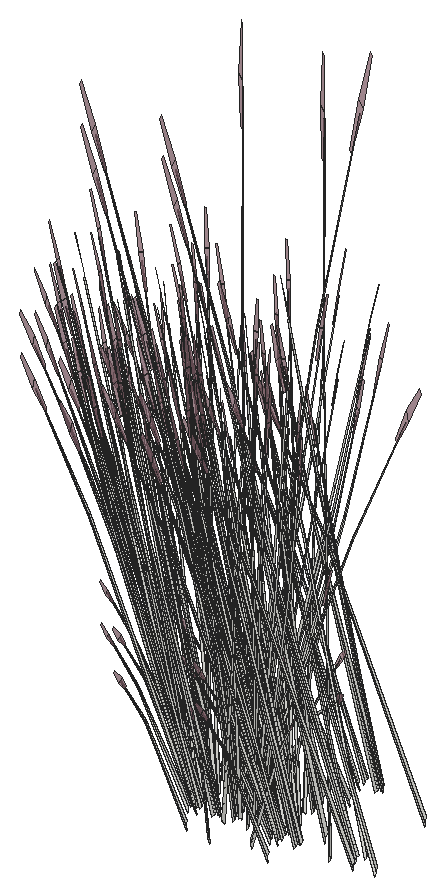
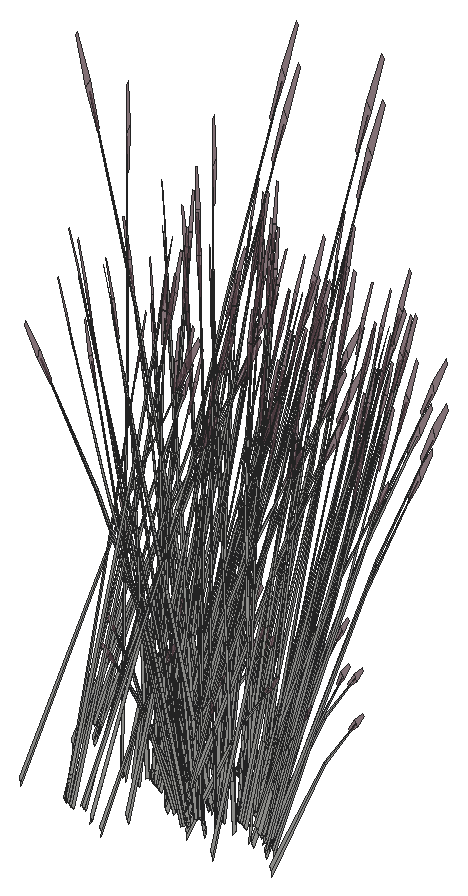
# SketchUp Ruby script. Lengths in inches.
U = 1.inch
M = Sketchup.active_model
def pt(a) = Geom::Point3d.new(a.map { |v| v * U })
def face(e, loops, mat)
  f = e.add_face(loops[0].map { |a| pt(a) })
  loops[1..].each { |l| e.add_face(l.map { |a| pt(a) }).erase! }
  f.material = f.back_material = mat if mat
  f
end
# faces: each face lists its corners as indices into pts; further lists are holes
def faces(e, pts, list, mat = nil) = list.each { |f| face(e, (f[0].is_a?(Array) ? f : [f]).map { |l| l.map { |i| pts[i] } }, mat) }
# xy, xz, yz: faces in a plane at the given z, y or x. An outline is a flat list of corners, or four numbers for a rectangle; further outlines are holes
def ring(l) = l.size == 4 ? [[l[0], l[1]], [l[2], l[1]], [l[2], l[3]], [l[0], l[3]]] : l.each_slice(2).to_a
def flat(e, list, mat, &to3) = list.each { |f| face(e, (f[0].is_a?(Array) ? f : [f]).map { |l| ring(l).map { |u, v| to3.(u, v) } }, mat) }
def xy(e, z, list, mat = nil) = flat(e, list, mat) { |x, y| [x, y, z] }
def xz(e, y, list, mat = nil) = flat(e, list, mat) { |x, z| [x, y, z] }
def yz(e, x, list, mat = nil) = flat(e, list, mat) { |y, z| [x, y, z] }
def lines(e, pts, list) = list.each { |a, b| e.add_line(pt(pts[a]), pt(pts[b])) }
# prism: a flat outline (further loops are holes) pulled along v
def prism(e, loops, v, mat = nil)
  f = face(e, loops, mat); d = Geom::Vector3d.new(v.map { |x| x * U })
  f.pushpull(f.normal.samedirection?(d) ? d.length : -d.length)
end
def box(e, o, s, mat = nil) = prism(e, [[o, [o[0] + s[0], o[1], o[2]], [o[0] + s[0], o[1] + s[1], o[2]], [o[0], o[1] + s[1], o[2]]]], [0, 0, s[2]], mat)
def at(x, y, z, deg = 0) = Geom::Transformation.translation(pt([x, y, z])) * Geom::Transformation.rotation(ORIGIN, Z_AXIS, deg.degrees)
def axes(o, x, y, z) = Geom::Transformation.new([*x, 0, *y, 0, *z, 0, *pt(o).to_a, 1])
def part(name) = M.definitions.add(name)
# library, detail: a bought-in or finely detailed component or shape, given as its bounding box
def library(name, o, s) = part(name).tap { |d| box(d.entities, o, s) }
def detail(e, o, s) = box(e.add_group.entities, o, s)
def put(e, d, t, mat = nil) = e.add_instance(d, t).tap { |i| i.material = mat if mat }
def group(e, t, mat = nil) = e.add_group.tap { |g| g.transformation = t; g.material = mat if mat }.entities
root = M.entities
M.materials.add("LightPink_Translucent").color = [144, 107, 117]
M.materials["LightPink_Translucent"].alpha = 0.75
c1 = part("blade")
p = [[2.15,0.21,22],[0,0.17,0],[0.09,0.45,0],[2.18,0.31,22],[2.29,0.31,22],[0.38,0.45,0],
  [2.48,0.24,33],[2.49,0.24,33],[2.48,0.22,33]]
faces(c1.entities,p,[[0,1,2,3],[4,5,2,3],[6,3,4,7],[8,0,3,6]])
c2 = part("seeds")
p = [[0.3,-0.1,1.38],[-0.01,-0.03,1.59],[-0.01,-0.03,0.03],[0.14,-0.07,-0.07],[0.29,-0.03,3],[0.15,0.01,3.11]]
faces(c2.entities,p,[[0,1,2,3],[1,0,4,5]],"LightPink_Translucent")
c3 = part("blade with seeds")
put(c3.entities,c1,at(0,0,0))
put(c3.entities,c2,axes([2.4,0.25,30.99],[1.5799,-0.05474,1.17369],[-0.12525,1.92788,0.29478],[-0.07173,-0.02425,1.56792]))
put(root,c3,axes([327.44,15.14,51.43],[0.11542,0.12546,1.51428],[-0.53333,0.10562,0.12244],[-0.12054,-0.19696,0.64734]))
put(root,c3,axes([333.1,15.14,51.43],[0.11542,0.12546,1.51428],[-0.53333,0.10562,0.12244],[-0.12054,-0.19696,0.64734]))
put(root,c3,axes([328.86,15.23,52.4],[-0.24099,-0.31773,-0.62776],[0.49607,-0.17707,0.07576],[-0.05635,-0.15352,0.88802]))
put(root,c3,axes([334.52,15.23,52.4],[-0.24099,-0.31773,-0.62776],[0.49607,-0.17707,0.07576],[-0.05635,-0.15352,0.88802]))
put(root,c3,axes([329.86,15.54,52.4],[0.01314,-0.36145,-0.62776],[0.55324,0.02428,0.07576],[0.05838,-0.15313,0.88802]))
put(root,c3,axes([328.91,14.96,52],[0.15222,-0.30049,-0.31292],[0.44409,0.08764,0.40398],[-0.04072,-0.12098,0.77298]))
put(root,c3,axes([329.24,15.36,51.43],[-0.09401,0.13431,1.51428],[-0.3944,-0.27795,0.12244],[0.17792,-0.17323,0.64734]))
put(root,c3,axes([328.68,15.17,52.14],[-0.49634,-0.09796,-0.45151],[0.17013,-0.33585,-0.34973],[-0.04551,-0.13522,0.86392]))
put(root,c3,axes([334.34,15.17,52.14],[-0.49634,-0.09796,-0.45151],[0.17013,-0.33585,-0.34973],[-0.04551,-0.13522,0.86392]))
put(root,c3,axes([328.99,14.33,50.44],[0.06477,0.22786,1.01491],[-0.35932,-0.1262,0.74569],[0.03867,-0.11667,0.22354]))
put(root,c3,axes([329.75,15.42,52.14],[-0.36145,-0.26255,-0.45151],[0.38183,-0.22994,-0.34973],[0.055,-0.1334,0.86392]))
put(root,c3,axes([329.11,15.15,52.45],[-0.49409,0.18193,-0.10745],[-0.24281,-0.32289,-0.59638],[-0.06519,-0.13607,0.90619]))
put(root,c3,axes([334.76,15.15,52.45],[-0.49409,0.18193,-0.10745],[-0.24281,-0.32289,-0.59638],[-0.06519,-0.13607,0.90619]))
put(root,c3,axes([330.13,15.56,52.45],[-0.55492,-0.01936,-0.10745],[0.01517,-0.36657,-0.59638],[0.03855,-0.14118,0.90619]))
put(root,c3,axes([330.09,15.32,52],[0.34164,-0.20573,-0.31292],[0.3234,0.23491,0.40398],[0.04921,-0.11936,0.77298]))
put(root,c3,axes([327.14,14.6,50.44],[0.26338,0.136,1.01491],[-0.38358,0.08175,0.74569],[-0.08207,-0.10452,0.22354]))
put(root,c3,axes([332.8,14.6,50.44],[0.26338,0.136,1.01491],[-0.38358,0.08175,0.74569],[-0.08207,-0.10452,0.22354]))
put(root,c3,axes([327.78,15.32,52.4],[-0.43054,-0.18887,-0.62776],[0.30598,-0.33097,0.07576],[-0.15599,-0.11277,0.88802]))
put(root,c3,axes([333.43,15.32,52.4],[-0.43054,-0.18887,-0.62776],[0.30598,-0.33097,0.07576],[-0.15599,-0.11277,0.88802]))
put(root,c3,axes([327.625,15.07,52],[-0.07798,-0.31474,-0.31292],[0.44579,-0.08311,0.40398],[-0.11974,-0.09019,0.77298]))
put(root,c3,axes([333.28,15.07,52],[-0.07798,-0.31474,-0.31292],[0.44579,-0.08311,0.40398],[-0.11974,-0.09019,0.77298]))
put(root,c3,axes([326.67,15.53,51.43],[0.18755,0.06732,1.51428],[-0.38813,0.28243,0.12244],[-0.24191,-0.12741,0.64734]))
put(root,c3,axes([332.32,15.53,51.43],[0.18755,0.06732,1.51428],[-0.38813,0.28243,0.12244],[-0.24191,-0.12741,0.64734]))
put(root,c3,axes([337.92,15.53,51.43],[0.18755,0.06732,1.51428],[-0.38813,0.28243,0.12244],[-0.24191,-0.12741,0.64734]))
put(root,c3,axes([327.57,15.33,52.14],[-0.49824,0.09289,-0.45151],[-0.08716,-0.35177,-0.34973],[-0.13382,-0.10081,0.86392]))
put(root,c3,axes([333.23,15.33,52.14],[-0.49824,0.09289,-0.45151],[-0.08716,-0.35177,-0.34973],[-0.13382,-0.10081,0.86392]))
put(root,c3,axes([330.52,16.17,52.4],[0.26374,-0.30832,-0.62776],[0.46217,0.21911,0.07576],[0.15748,-0.11171,0.88802]))
put(root,c3,axes([330.5,16.03,52.14],[-0.12971,-0.3568,-0.45151],[0.49122,-0.06241,-0.34973],[0.14077,-0.09583,0.86392]))
put(root,c3,axes([330.74,16.28,52.45],[-0.46706,-0.21546,-0.10745],[0.26908,-0.31203,-0.59638],[0.13196,-0.10846,0.90619]))
put(root,c3,axes([328.81,17.46,50.9375],[0.43633,0.15757,1.33654],[-0.42745,0.33945,0.52853],[-0.19146,-0.20119,1.12046]))
put(root,c3,axes([334.46,17.46,50.9375],[0.43633,0.15757,1.33654],[-0.42745,0.33945,0.52853],[-0.19146,-0.20119,1.12046]))
put(root,c3,axes([331.11,15.32,50.44],[-0.16818,0.19891,1.01491],[-0.14456,-0.26725,0.74569],[0.1389,-0.06697,0.22354]))
put(root,c3,axes([330.87,16.0625,52],[0.43951,-0.05584,-0.31292],[0.11606,0.31924,0.40398],[0.12595,-0.08575,0.77298]))
put(root,c3,axes([326.59,15.625,52],[-0.28729,-0.24465,-0.31292],[0.32804,-0.23159,0.40398],[-0.16667,-0.03524,0.77298]))
put(root,c3,axes([332.25,15.625,52],[-0.28729,-0.24465,-0.31292],[0.32804,-0.23159,0.40398],[-0.16667,-0.03524,0.77298]))
put(root,c3,axes([326.9,15.79,52.4],[-0.50473,-0.00941,-0.62776],[0.0339,-0.39618,0.07576],[-0.21383,-0.04181,0.88802]))
put(root,c3,axes([332.55,15.79,52.4],[-0.50473,-0.00941,-0.62776],[0.0339,-0.39618,0.07576],[-0.21383,-0.04181,0.88802]))
put(root,c3,axes([338.15,15.79,52.4],[-0.50473,-0.00941,-0.62776],[0.0339,-0.39618,0.07576],[-0.21383,-0.04181,0.88802]))
put(root,c3,axes([330.24,18.54,51.43],[0.11542,0.12546,1.51428],[-0.53333,0.10562,0.12244],[-0.12054,-0.19696,0.64734]))
put(root,c3,axes([331.66,18.63,52.4],[-0.24099,-0.31773,-0.62776],[0.49607,-0.17707,0.07576],[-0.05635,-0.15352,0.88802]))
put(root,c3,axes([326.73,15.87,52.14],[-0.36663,0.25884,-0.45151],[-0.32109,-0.27343,-0.34973],[-0.18628,-0.03938,0.86392]))
put(root,c3,axes([332.39,15.87,52.14],[-0.36663,0.25884,-0.45151],[-0.32109,-0.27343,-0.34973],[-0.18628,-0.03938,0.86392]))
put(root,c3,axes([324.42,18.85,51.43],[0.11542,0.12546,1.51428],[-0.53333,0.10562,0.12244],[-0.12054,-0.19696,0.64734]))
put(root,c3,axes([325.9,16.21,50.44],[0.32236,-0.02796,1.01491],[-0.20448,0.24636,0.74569],[-0.1593,-0.03696,0.22354]))
put(root,c3,axes([331.5625,16.21,50.44],[0.32236,-0.02796,1.01491],[-0.20448,0.24636,0.74569],[-0.1593,-0.03696,0.22354]))
put(root,c3,axes([325.84,18.9375,52.4],[-0.24099,-0.31773,-0.62776],[0.49607,-0.17707,0.07576],[-0.05635,-0.15352,0.88802]))
put(root,c3,axes([326.92,15.6,52.45],[-0.02704,0.39739,-0.10745],[-0.51189,-0.01086,-0.59638],[-0.19715,-0.0276,0.90619]))
put(root,c3,axes([332.58,15.6,52.45],[-0.02704,0.39739,-0.10745],[-0.51189,-0.01086,-0.59638],[-0.19715,-0.0276,0.90619]))
put(root,c3,axes([331.7,18.36,52],[0.15222,-0.30049,-0.31292],[0.44409,0.08764,0.40398],[-0.04072,-0.12098,0.77298]))
put(root,c3,axes([326.27,16.14,51.43],[0.20943,-0.00885,1.51428],[-0.13893,0.38357,0.12244],[-0.29846,-0.02372,0.64734]))
put(root,c3,axes([331.93,16.14,51.43],[0.20943,-0.00885,1.51428],[-0.13893,0.38357,0.12244],[-0.29846,-0.02372,0.64734]))
put(root,c3,axes([337.52,16.14,51.43],[0.20943,-0.00885,1.51428],[-0.13893,0.38357,0.12244],[-0.29846,-0.02372,0.64734]))
put(root,c3,axes([331.48,18.57,52.14],[-0.49634,-0.09796,-0.45151],[0.17013,-0.33585,-0.34973],[-0.04551,-0.13522,0.86392]))
put(root,c3,axes([331.78,17.73,50.44],[0.06477,0.22786,1.01491],[-0.35932,-0.1262,0.74569],[0.03867,-0.11667,0.22354]))
put(root,c3,axes([326.84,19.25,52.4],[0.01314,-0.36145,-0.62776],[0.55324,0.02428,0.07576],[0.05838,-0.15313,0.88802]))
put(root,c3,axes([332.55,18.82,52.14],[-0.36145,-0.26255,-0.45151],[0.38183,-0.22994,-0.34973],[0.055,-0.1334,0.86392]))
put(root,c3,axes([325.89,18.67,52],[0.15222,-0.30049,-0.31292],[0.44409,0.08764,0.40398],[-0.04072,-0.12098,0.77298]))
put(root,c3,axes([326.22,19.07,51.43],[-0.09401,0.13431,1.51428],[-0.3944,-0.27795,0.12244],[0.17792,-0.17323,0.64734]))
put(root,c3,axes([325.66,18.875,52.14],[-0.49634,-0.09796,-0.45151],[0.17013,-0.33585,-0.34973],[-0.04551,-0.13522,0.86392]))
put(root,c3,axes([325.97,18.03,50.44],[0.06477,0.22786,1.01491],[-0.35932,-0.1262,0.74569],[0.03867,-0.11667,0.22354]))
put(root,c3,axes([331.9,18.55,52.45],[-0.49409,0.18193,-0.10745],[-0.24281,-0.32289,-0.59638],[-0.06519,-0.13607,0.90619]))
put(root,c3,axes([326.73,19.13,52.14],[-0.36145,-0.26255,-0.45151],[0.38183,-0.22994,-0.34973],[0.055,-0.1334,0.86392]))
put(root,c3,axes([332.93,18.96,52.45],[-0.55492,-0.01936,-0.10745],[0.01517,-0.36657,-0.59638],[0.03855,-0.14118,0.90619]))
put(root,c3,axes([329.9375,18,50.44],[0.26338,0.136,1.01491],[-0.38358,0.08175,0.74569],[-0.08207,-0.10452,0.22354]))
put(root,c3,axes([330.57,18.72,52.4],[-0.43054,-0.18887,-0.62776],[0.30598,-0.33097,0.07576],[-0.15599,-0.11277,0.88802]))
put(root,c3,axes([330.42,18.47,52],[-0.07798,-0.31474,-0.31292],[0.44579,-0.08311,0.40398],[-0.11974,-0.09019,0.77298]))
put(root,c3,axes([326.08,18.86,52.45],[-0.49409,0.18193,-0.10745],[-0.24281,-0.32289,-0.59638],[-0.06519,-0.13607,0.90619]))
put(root,c3,axes([327.11,19.27,52.45],[-0.55492,-0.01936,-0.10745],[0.01517,-0.36657,-0.59638],[0.03855,-0.14118,0.90619]))
put(root,c3,axes([327.07,19.03,52],[0.34164,-0.20573,-0.31292],[0.3234,0.23491,0.40398],[0.04921,-0.11936,0.77298]))
put(root,c3,axes([324.12,18.31,50.44],[0.26338,0.136,1.01491],[-0.38358,0.08175,0.74569],[-0.08207,-0.10452,0.22354]))
put(root,c3,axes([324.75,19.03,52.4],[-0.43054,-0.18887,-0.62776],[0.30598,-0.33097,0.07576],[-0.15599,-0.11277,0.88802]))
put(root,c3,axes([324.61,18.78,52],[-0.07798,-0.31474,-0.31292],[0.44579,-0.08311,0.40398],[-0.11974,-0.09019,0.77298]))
put(root,c3,axes([329.46,18.93,51.43],[0.18755,0.06732,1.51428],[-0.38813,0.28243,0.12244],[-0.24191,-0.12741,0.64734]))
put(root,c3,axes([326.09,16.47,52],[-0.41962,-0.10901,-0.31292],[0.12239,-0.31802,0.40398],[-0.16894,0.02916,0.77298]))
put(root,c3,axes([331.74,16.47,52],[-0.41962,-0.10901,-0.31292],[0.12239,-0.31802,0.40398],[-0.16894,0.02916,0.77298]))
put(root,c3,axes([337.34,16.47,52],[-0.41962,-0.10901,-0.31292],[0.12239,-0.31802,0.40398],[-0.16894,0.02916,0.77298]))
put(root,c3,axes([330.37,18.73,52.14],[-0.49824,0.09289,-0.45151],[-0.08716,-0.35177,-0.34973],[-0.13382,-0.10081,0.86392]))
put(root,c3,axes([323.65,19.24,51.43],[0.18755,0.06732,1.51428],[-0.38813,0.28243,0.12244],[-0.24191,-0.12741,0.64734]))
put(root,c3,axes([324.55,19.04,52.14],[-0.49824,0.09289,-0.45151],[-0.08716,-0.35177,-0.34973],[-0.13382,-0.10081,0.86392]))
put(root,c3,axes([327.37,16.42,50.95],[0.14352,-0.05653,1.56454],[0.04949,0.39467,0.12244],[-0.31087,0.05237,0.55918]))
put(root,c3,axes([333.02,16.42,50.95],[0.14352,-0.05653,1.56454],[0.04949,0.39467,0.12244],[-0.31087,0.05237,0.55918]))
put(root,c3,axes([338.62,16.42,50.95],[0.14352,-0.05653,1.56454],[0.04949,0.39467,0.12244],[-0.31087,0.05237,0.55918]))
put(root,c3,axes([327.5,19.88,52.4],[0.26374,-0.30832,-0.62776],[0.46217,0.21911,0.07576],[0.15748,-0.11171,0.88802]))
put(root,c3,axes([327.48,19.73,52.14],[-0.12971,-0.3568,-0.45151],[0.49122,-0.06241,-0.34973],[0.14077,-0.09583,0.86392]))
put(root,c3,axes([331.6,20.86,50.9375],[0.43633,0.15757,1.33654],[-0.42745,0.33945,0.52853],[-0.19146,-0.20119,1.12046]))
put(root,c3,axes([327.71,19.99,52.45],[-0.46706,-0.21546,-0.10745],[0.26908,-0.31203,-0.59638],[0.13196,-0.10846,0.90619]))
put(root,c3,axes([326.375,16.64,52.14],[-0.13679,0.35544,-0.45151],[-0.46898,-0.12183,-0.34973],[-0.18882,0.03259,0.86392]))
put(root,c3,axes([332.03,16.64,52.14],[-0.13679,0.35544,-0.45151],[-0.46898,-0.12183,-0.34973],[-0.18882,0.03259,0.86392]))
put(root,c3,axes([326.35,16.33,52.45],[0.25405,0.35383,-0.10745],[-0.45089,0.17388,-0.59638],[-0.19001,0.04668,0.90619]))
put(root,c3,axes([332.01,16.33,52.45],[0.25405,0.35383,-0.10745],[-0.45089,0.17388,-0.59638],[-0.19001,0.04668,0.90619]))
put(root,c3,axes([331.37,17.87,51.47],[-0.09664,-0.32847,-0.03085],[0.45676,-0.07551,-0.13989],[0.09538,0.02082,0.4614]))
put(root,c3,axes([325.78,21.17,50.9375],[0.43633,0.15757,1.33654],[-0.42745,0.33945,0.52853],[-0.19146,-0.20119,1.12046]))
put(root,c3,axes([329.39,19.02,52],[-0.28729,-0.24465,-0.31292],[0.32804,-0.23159,0.40398],[-0.16667,-0.03524,0.77298]))
put(root,c3,axes([328.09,19.02,50.44],[-0.16818,0.19891,1.01491],[-0.14456,-0.26725,0.74569],[0.1389,-0.06697,0.22354]))
put(root,c3,axes([327.84,19.77,52],[0.43951,-0.05584,-0.31292],[0.11606,0.31924,0.40398],[0.12595,-0.08575,0.77298]))
put(root,c3,axes([323.57,19.33,52],[-0.28729,-0.24465,-0.31292],[0.32804,-0.23159,0.40398],[-0.16667,-0.03524,0.77298]))
put(root,c3,axes([329.69,19.1875,52.4],[-0.50473,-0.00941,-0.62776],[0.0339,-0.39618,0.07576],[-0.21383,-0.04181,0.88802]))
put(root,c3,axes([326.36,16.82,51.43],[0.17519,-0.08265,1.51428],[0.14749,0.38193,0.12244],[-0.27504,0.08632,0.64734]))
put(root,c3,axes([332.01,16.82,51.43],[0.17519,-0.08265,1.51428],[0.14749,0.38193,0.12244],[-0.27504,0.08632,0.64734]))
put(root,c3,axes([337.61,16.82,51.43],[0.17519,-0.08265,1.51428],[0.14749,0.38193,0.12244],[-0.27504,0.08632,0.64734]))
put(root,c3,axes([323.875,19.5,52.4],[-0.50473,-0.00941,-0.62776],[0.0339,-0.39618,0.07576],[-0.21383,-0.04181,0.88802]))
put(root,c3,axes([329.11,20.28,52.17],[0.07006,-0.05952,1.54581],[-0.08968,-0.3651,-0.24447],[0.1758,-0.06922,0.12397]))
put(root,c3,axes([325.45,18.16,50.44],[0.21042,-0.1771,1.01491],[0.08303,0.28036,0.74569],[-0.15207,0.0502,0.22354]))
put(root,c3,axes([331.1,18.16,50.44],[0.21042,-0.1771,1.01491],[0.08303,0.28036,0.74569],[-0.15207,0.0502,0.22354]))
put(root,c3,axes([329.53,19.27,52.14],[-0.36663,0.25884,-0.45151],[-0.32109,-0.27343,-0.34973],[-0.18628,-0.03938,0.86392]))
put(root,c3,axes([328.7,19.61,50.44],[0.32236,-0.02796,1.01491],[-0.20448,0.24636,0.74569],[-0.1593,-0.03696,0.22354]))
put(root,c3,axes([326.24,17.39,52],[-0.43951,0.05584,-0.31292],[-0.11606,-0.31924,0.40398],[-0.12595,0.08575,0.77298]))
put(root,c3,axes([331.9,17.39,52],[-0.43951,0.05584,-0.31292],[-0.11606,-0.31924,0.40398],[-0.12595,0.08575,0.77298]))
put(root,c3,axes([329.72,19,52.45],[-0.02704,0.39739,-0.10745],[-0.51189,-0.01086,-0.59638],[-0.19715,-0.0276,0.90619]))
put(root,c3,axes([323.71,19.58,52.14],[-0.36663,0.25884,-0.45151],[-0.32109,-0.27343,-0.34973],[-0.18628,-0.03938,0.86392]))
put(root,c3,axes([329.07,19.54,51.43],[0.20943,-0.00885,1.51428],[-0.13893,0.38357,0.12244],[-0.29846,-0.02372,0.64734]))
put(root,c3,axes([322.88,19.92,50.44],[0.32236,-0.02796,1.01491],[-0.20448,0.24636,0.74569],[-0.1593,-0.03696,0.22354]))
put(root,c3,axes([329.48,17.2,51.43],[-0.18755,-0.06732,1.51428],[0.38813,-0.28243,0.12244],[0.24191,0.12741,0.64734]))
put(root,c3,axes([332.69,22.73,51.43],[0.11542,0.12546,1.51428],[-0.53333,0.10562,0.12244],[-0.12054,-0.19696,0.64734]))
put(root,c3,axes([323.9,19.31,52.45],[-0.02704,0.39739,-0.10745],[-0.51189,-0.01086,-0.59638],[-0.19715,-0.0276,0.90619]))
put(root,c3,axes([329.52,16.32,51.95],[-0.4363,-0.20303,1.22187],[0.46069,-0.31611,0.5272],[0.14077,0.1905,1.18105]))
put(root,c3,axes([327.73,20.83,52.45],[-0.25405,-0.35383,-0.10745],[0.45089,-0.17388,-0.59638],[0.19001,-0.04668,0.90619]))
put(root,c3,axes([327.71,20.53,52.14],[0.13679,-0.35544,-0.45151],[0.46898,0.12183,-0.34973],[0.18882,-0.03259,0.86392]))
put(root,c3,axes([323.25,19.85,51.43],[0.20943,-0.00885,1.51428],[-0.13893,0.38357,0.12244],[-0.29846,-0.02372,0.64734]))
put(root,c3,axes([326.37,17.17,52.45],[0.46706,0.21546,-0.10745],[-0.26908,0.31203,-0.59638],[-0.13196,0.10846,0.90619]))
put(root,c3,axes([332.03,17.17,52.45],[0.46706,0.21546,-0.10745],[-0.26908,0.31203,-0.59638],[-0.13196,0.10846,0.90619]))
put(root,c3,axes([330.17,17.97,50.44],[-0.28429,-0.11236,1.01491],[0.36709,-0.11416,0.74569],[0.09901,0.0967,0.22354]))
put(root,c3,axes([334.11,22.83,52.4],[-0.24099,-0.31773,-0.62776],[0.49607,-0.17707,0.07576],[-0.05635,-0.15352,0.88802]))
put(root,c3,axes([329.18,18.29,52.45],[0.30087,-0.33447,-0.10745],[0.43572,0.19269,-0.59638],[0.15146,0.0945,0.90619]))
put(root,c3,axes([327,17.08,51.43],[0.12611,-0.12006,1.51428],[0.31843,0.32408,0.12244],[-0.2184,0.14759,0.64734]))
put(root,c3,axes([332.66,17.08,51.43],[0.12611,-0.12006,1.51428],[0.31843,0.32408,0.12244],[-0.2184,0.14759,0.64734]))
put(root,c3,axes([337.92,21.8,51.43],[0.18755,0.06732,1.51428],[-0.38813,0.28243,0.12244],[-0.24191,-0.12741,0.64734]))
put(root,c3,axes([326.6,17.43,52.14],[0.12971,0.3568,-0.45151],[-0.49122,0.06241,-0.34973],[-0.14077,0.09583,0.86392]))
put(root,c3,axes([332.26,17.43,52.14],[0.12971,0.3568,-0.45151],[-0.49122,0.06241,-0.34973],[-0.14077,0.09583,0.86392]))
put(root,c3,axes([327.62,20.66,52.4],[0.44368,-0.17257,-0.62776],[0.24726,0.35524,0.07576],[0.21437,-0.04035,0.88802]))
put(root,c3,axes([329.48,16.7,50.51],[-0.01379,-0.36791,1.24828],[0.62424,0.09537,0.52853],[-0.14764,0.20132,1.17828]))
put(root,c3,axes([335.14,16.7,50.51],[-0.01379,-0.36791,1.24828],[0.62424,0.09537,0.52853],[-0.14764,0.20132,1.17828]))
put(root,c3,axes([329.53,18.125,52.14],[0.49824,-0.09289,-0.45151],[0.08716,0.35177,-0.34973],[0.13382,0.10081,0.86392]))
put(root,c3,axes([334.16,22.56,52],[0.15222,-0.30049,-0.31292],[0.44409,0.08764,0.40398],[-0.04072,-0.12098,0.77298]))
put(root,c3,axes([333.93,22.76,52.14],[-0.49634,-0.09796,-0.45151],[0.17013,-0.33585,-0.34973],[-0.04551,-0.13522,0.86392]))
put(root,c3,axes([328.88,19.875,52],[-0.41962,-0.10901,-0.31292],[0.12239,-0.31802,0.40398],[-0.16894,0.02916,0.77298]))
put(root,c3,axes([326.91,17.37,51.43],[0.09401,-0.13431,1.51428],[0.3944,0.27795,0.12244],[-0.17792,0.17323,0.64734]))
put(root,c3,axes([332.5625,17.37,51.43],[0.09401,-0.13431,1.51428],[0.3944,0.27795,0.12244],[-0.17792,0.17323,0.64734]))
put(root,c3,axes([328,20.6875,52],[0.41962,0.10901,-0.31292],[-0.12239,0.31802,0.40398],[0.16894,-0.02916,0.77298]))
put(root,c3,axes([334.36,22.75,52.45],[-0.49409,0.18193,-0.10745],[-0.24281,-0.32289,-0.59638],[-0.06519,-0.13607,0.90619]))
put(root,c3,axes([323.07,20.18,52],[-0.41962,-0.10901,-0.31292],[0.12239,-0.31802,0.40398],[-0.16894,0.02916,0.77298]))
put(root,c3,axes([332.39,22.2,50.44],[0.26338,0.136,1.01491],[-0.38358,0.08175,0.74569],[-0.08207,-0.10452,0.22354]))
put(root,c3,axes([333.03,22.92,52.4],[-0.43054,-0.18887,-0.62776],[0.30598,-0.33097,0.07576],[-0.15599,-0.11277,0.88802]))
put(root,c3,axes([327.01,18.13,52],[-0.34164,0.20573,-0.31292],[-0.3234,-0.23491,0.40398],[-0.04921,0.11936,0.77298]))
put(root,c3,axes([332.67,18.13,52],[-0.34164,0.20573,-0.31292],[-0.3234,-0.23491,0.40398],[-0.04921,0.11936,0.77298]))
put(root,c3,axes([332.88,22.67,52],[-0.07798,-0.31474,-0.31292],[0.44579,-0.08311,0.40398],[-0.11974,-0.09019,0.77298]))
put(root,c3,axes([328,18.3,52.45],[0.49409,-0.18193,-0.10745],[0.24281,0.32289,-0.59638],[0.06519,0.13607,0.90619]))
put(root,c3,axes([327.23,18.93,50.44],[-0.01307,-0.23234,1.01491],[0.32652,0.16572,0.74569],[-0.06422,0.11074,0.22354]))
